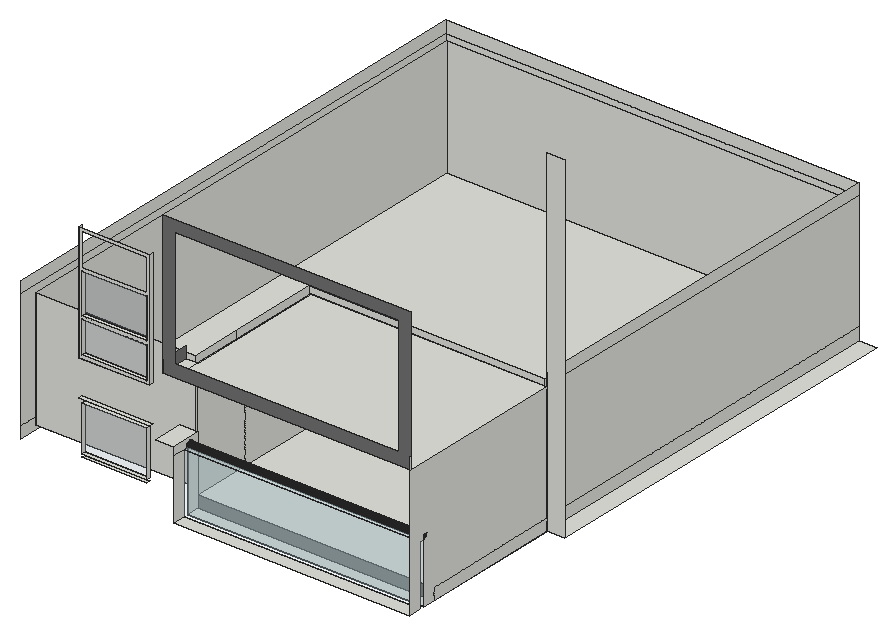
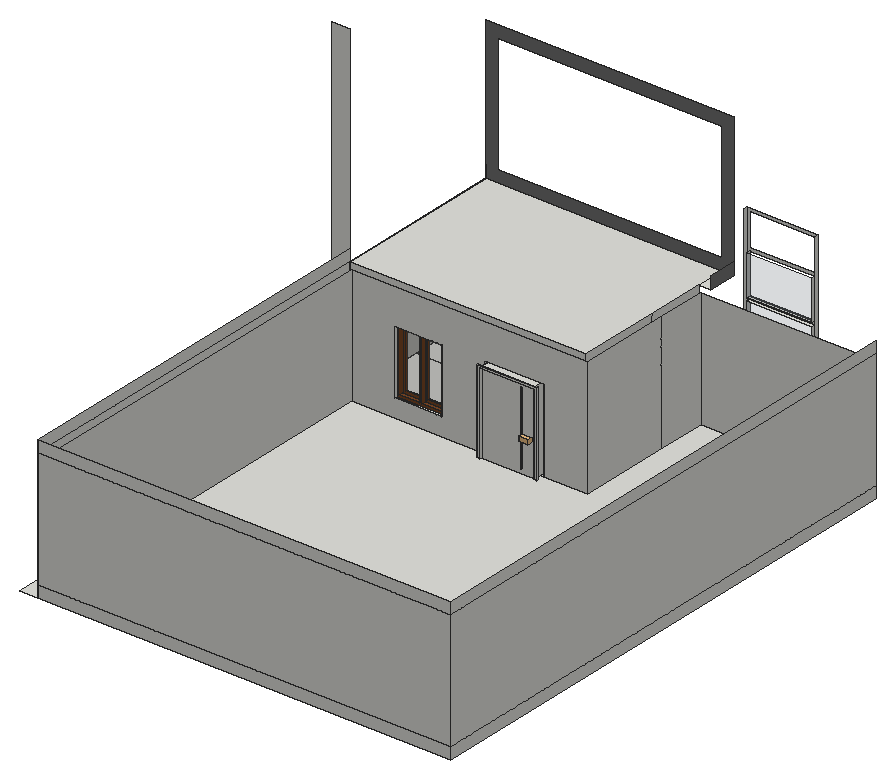
# SketchUp Ruby script. Lengths in inches.
U = 1.inch
M = Sketchup.active_model
def pt(a) = Geom::Point3d.new(a.map { |v| v * U })
def face(e, loops, mat)
  f = e.add_face(loops[0].map { |a| pt(a) })
  loops[1..].each { |l| e.add_face(l.map { |a| pt(a) }).erase! }
  f.material = f.back_material = mat if mat
  f
end
# faces: each face lists its corners as indices into pts; further lists are holes
def faces(e, pts, list, mat = nil) = list.each { |f| face(e, (f[0].is_a?(Array) ? f : [f]).map { |l| l.map { |i| pts[i] } }, mat) }
# xy, xz, yz: faces in a plane at the given z, y or x. An outline is a flat list of corners, or four numbers for a rectangle; further outlines are holes
def ring(l) = l.size == 4 ? [[l[0], l[1]], [l[2], l[1]], [l[2], l[3]], [l[0], l[3]]] : l.each_slice(2).to_a
def flat(e, list, mat, &to3) = list.each { |f| face(e, (f[0].is_a?(Array) ? f : [f]).map { |l| ring(l).map { |u, v| to3.(u, v) } }, mat) }
def xy(e, z, list, mat = nil) = flat(e, list, mat) { |x, y| [x, y, z] }
def xz(e, y, list, mat = nil) = flat(e, list, mat) { |x, z| [x, y, z] }
def yz(e, x, list, mat = nil) = flat(e, list, mat) { |y, z| [x, y, z] }
def lines(e, pts, list) = list.each { |a, b| e.add_line(pt(pts[a]), pt(pts[b])) }
# prism: a flat outline (further loops are holes) pulled along v
def prism(e, loops, v, mat = nil)
  f = face(e, loops, mat); d = Geom::Vector3d.new(v.map { |x| x * U })
  f.pushpull(f.normal.samedirection?(d) ? d.length : -d.length)
end
def box(e, o, s, mat = nil) = prism(e, [[o, [o[0] + s[0], o[1], o[2]], [o[0] + s[0], o[1] + s[1], o[2]], [o[0], o[1] + s[1], o[2]]]], [0, 0, s[2]], mat)
def at(x, y, z, deg = 0) = Geom::Transformation.translation(pt([x, y, z])) * Geom::Transformation.rotation(ORIGIN, Z_AXIS, deg.degrees)
def axes(o, x, y, z) = Geom::Transformation.new([*x, 0, *y, 0, *z, 0, *pt(o).to_a, 1])
def part(name) = M.definitions.add(name)
# library, detail: a bought-in or finely detailed component or shape, given as its bounding box
def library(name, o, s) = part(name).tap { |d| box(d.entities, o, s) }
def detail(e, o, s) = box(e.add_group.entities, o, s)
def put(e, d, t, mat = nil) = e.add_instance(d, t).tap { |i| i.material = mat if mat }
def group(e, t, mat = nil) = e.add_group.tap { |g| g.transformation = t; g.material = mat if mat }.entities
root = M.entities
M.materials.add("Glass_Basic_01").color = [161, 173, 186]
M.materials["Glass_Basic_01"].alpha = 0.25
M.materials.add("Glass_Safety_01").color = [204, 235, 244]
M.materials["Glass_Safety_01"].alpha = 0.25
M.materials.add("M05_Graphite_Haze").color = [114, 114, 114]
M.materials.add("Metal_06_1K").color = [238, 236, 231]
M.materials.add("[Translucent Glass Gray]").color = [132, 132, 132]
M.materials["[Translucent Glass Gray]"].alpha = 0.25
M.materials.add("[Wood Veneer 01]").color = [120, 70, 37]
c1 = part("Group\#8")
xy(c1.entities,0,[[0,0,19.69,1.18]],"[Wood Veneer 01]")
xy(c1.entities,2.76,[[2.76,0,16.93,1.18]],"[Wood Veneer 01]")
xy(c1.entities,60.24,[[2.76,0,16.93,1.18]],"[Wood Veneer 01]")
xy(c1.entities,62.99,[[0,0,19.69,1.18]],"[Wood Veneer 01]")
xz(c1.entities,0,[[2.76,2.76,16.93,60.24]],"[Translucent Glass Gray]")
xz(c1.entities,0,[[[0,0,19.69,62.99],[2.76,2.76,16.93,60.24]]],"[Wood Veneer 01]")
xz(c1.entities,1.18,[[[0,0,19.69,62.99],[2.76,2.76,16.93,60.24]]],"[Wood Veneer 01]")
yz(c1.entities,0,[[0,0,1.18,62.99]],"[Wood Veneer 01]")
yz(c1.entities,2.76,[[0,2.76,1.18,60.24]],"[Wood Veneer 01]")
yz(c1.entities,16.93,[[0,2.76,1.18,60.24]],"[Wood Veneer 01]")
yz(c1.entities,19.69,[[0,0,1.18,62.99]],"[Wood Veneer 01]")
c2 = part("pintu 2")
put(c2.entities,c1,at(-19.69,0,1.97))
g1 = group(c2.entities,at(-21.65,0,0))
prism(g1,[[[0,0,66.93],[0,0,0],[45.28,0,0],[45.28,0,66.93]],[[43.31,0,1.97],[23.62,0,1.97],[23.62,0,64.96],[43.31,0,64.96]],[[21.65,0,64.96],[21.65,0,1.97],[1.97,0,1.97],[1.97,0,64.96]]],[0,5.91,0],"[Wood Veneer 01]")
put(c2.entities,c1,at(1.97,0,1.97))
c3 = library("CLASSIC-BRASS_CHAUTAUQUA_LEVER-HARDWARE",[7.77,-2.58,0],[5.5,6.97,4.76])
xy(root,144,[[271.5,47.44,511.5,60.19],[271.5,64.66,511.5,77.44],[271.5,77.44,511.5,221.44],[511.5,221.87,529.5,617.44]])
xy(root,152.13,[[157.5,73.44,223.5,77.44]])
xy(root,155,[[157.5,73.44,223.5,77.44]])
xy(root,156,[[271.5,77.44,511.5,137.44],[100.5,86.44,262.5,86.44,262.5,230.44,310.875,230.44,310.875,233.83,310.2,233.83,310.2,237.47,307.5,237.47,307.5,238.93,310.875,238.93,310.875,233.83,311.21,233.83,311.21,237.47,364.86,237.47,364.86,238.93,368.23,238.93,368.23,237.47,365.53,237.47,365.53,233.83,364.86,233.83,364.86,230.44,502.5,230.44,502.5,608.44,100.5,608.44],[271.5,137.44,511.5,137.44,511.5,221.44,364.86,221.44,364.86,222.9,364.52,222.9,364.52,230.44,311.21,230.44,311.21,222.9,310.875,222.9,310.875,221.44,271.5,221.44],[307.5,221.44,310.875,222.9],[364.86,221.44,367.5,222.9],
  [367.5,221.44,368.23,222.9],[307.5,222.9,310.875,230.44],[310.875,222.9,311.21,230.44],[364.52,222.9,364.86,230.44],[364.86,222.9,367.5,230.44],
  [310.875,230.44,311.21,230.44,311.21,233.83,310.875,233.83,310.875,237.47,310.2,237.47,310.2,233.83,310.875,233.83],[311.21,230.44,364.52,233.83],[364.52,230.44,364.86,231.64],[364.52,231.64,364.86,231.64,364.86,233.83,365.2,233.83,365.2,237.47,364.86,237.47,364.86,233.83,364.52,233.83],[311.21,233.83,364.86,237.47],
  [365.2,233.83,365.53,237.47],[307.5,237.47,310.875,238.93],[364.86,237.47,368.23,238.93]])
xy(root,159.82,[[324.03,233.83,324.71,234.56],[324.03,236.75,324.71,237.47]])
xy(root,174.39,[[410.69,221.44,458.69,230.44]])
xy(root,202.13,[[157.5,73.44,223.5,77.44]])
xy(root,205.13,[[154.5,73.44,226.5,77.44]])
xy(root,205.15,[[271.5,60.19,511.5,64.66]],"Glass_Safety_01")
xy(root,213.3,[[253.5,47.44,271.5,77.44]])
xy(root,234.27,[[324.03,233.83,324.71,234.56],[324.03,236.75,324.71,237.47]])
xy(root,237.9,[[311.21,222.9,364.52,233.83]])
xy(root,238.09,[[310.875,221.44,364.86,222.9],[364.52,222.9,364.86,231.64],[310.2,233.83,310.875,237.47],[310.875,233.83,311.21,237.47],[311.21,233.83,364.86,237.47],
  [364.86,233.83,365.2,237.47],[365.2,233.83,365.53,237.47],[310.875,237.47,364.86,238.93]])
xy(root,239.43,[[310.875,222.9,364.86,237.47]])
xy(root,240,[[307.5,221.44,367.5,222.9],[367.5,221.44,368.23,222.9],[410.69,221.44,458.69,230.44],[307.5,222.9,367.5,230.44],[307.5,237.47,368.23,238.93]])
xy(root,242.1,[[154.5,73.44,226.5,77.44]])
xy(root,245.1,[[157.5,73.44,223.5,77.44]])
xy(root,276,[[259.5,48.44,271.5,77.44],[271.5,48.44,511.5,221.44]])
xy(root,278.1,[[157.5,73.44,223.5,77.44]])
xy(root,281.1,[[157.5,73.44,223.5,77.44]])
xz(root,48.44,[[[259.5,276,511.5,420],[271.5,288,499.5,408]]],"M05_Graphite_Haze")
xz(root,60.19,[[271.5,144,511.5,205.15]],"Glass_Safety_01")
xz(root,64.66,[[271.5,144,511.5,205.15]],"Glass_Safety_01")
xz(root,73.44,[[[154.5,242.1,226.5,361.04],[157.5,281.1,223.5,322.04],[157.5,325.04,223.5,358.04],[157.5,245.1,223.5,278.1]]])
xz(root,77.44,[[157.5,155,223.5,202.13],[157.5,245.1,223.5,278.1],[157.5,281.1,223.5,322.04]],"Glass_Basic_01")
xz(root,77.44,[[271.5,144,511.5,156]],"M05_Graphite_Haze")
xz(root,86.44,[[100.5,156,262.5,276]])
xz(root,221.44,[[[271.5,156,307.5,156,307.5,240,368.23,240,368.23,156,511.5,156,511.5,276,271.5,276],[410.69,174.39,458.69,240]],[307.5,156,310.875,156,310.875,238.09,364.86,238.09,364.86,156,367.5,156,367.5,240,307.5,240],[367.5,156,368.23,240]])
xz(root,221.87,[[511.5,144,529.5,488.3125]])
xz(root,222.9,[[307.5,156,310.875,238.47],[310.875,156,311.21,238.09],[364.52,156,364.86,238.09],[364.86,156,368.23,238.47],[311.21,237.9,364.52,238.09],
  [310.875,238.09,364.86,239.43],[307.5,238.47,307.5,240,368.23,240,368.23,238.47,364.86,238.47,364.86,239.43,310.875,239.43,310.875,238.47]])
xz(root,230.44,[[[262.5,156,262.5,276,502.5,276,502.5,156,367.5,156,367.5,240,307.5,240,307.5,156],[410.69,174.39,458.69,240]]])
xz(root,233.83,[[310.2,156,310.875,238.09],[310.875,156,311.21,237.9],[[311.21,156,364.52,237.9],[324.03,159.82,324.71,234.27]],[364.52,156,364.86,237.9],[364.86,156,365.2,238.09],
  [365.2,156,365.53,238.09],[310.875,237.9,311.21,238.09],[311.21,237.9,364.86,238.09]])
xz(root,234.56,[[324.03,159.82,324.71,234.27]])
xz(root,236.75,[[324.03,159.82,324.71,234.27]])
xz(root,237.47,[[307.5,156,310.2,156,310.2,238.09,310.875,238.09,310.875,238.47,307.5,238.47],[310.2,156,310.875,238.09],[[311.21,156,364.86,238.09],[324.03,159.82,324.71,234.27]],[364.86,156,365.2,238.09],[365.53,156,368.23,156,368.23,238.47,364.86,238.47,364.86,238.09,365.53,238.09],
  [365.2,156,365.53,238.09],[310.875,238.09,364.86,239.43],[307.5,238.47,310.875,238.47,310.875,239.43,364.86,239.43,364.86,238.47,368.23,238.47,368.23,240,307.5,240]])
xz(root,238.93,[[307.5,156,307.5,240,368.23,240,368.23,156,364.86,156,364.86,238.09,310.875,238.09,310.875,156]])
xz(root,608.44,[[100.5,156,502.5,276]])
xz(root,617.44,[[91.5,144,511.5,156],[91.5,156,511.5,276],[91.5,276,511.5,288]])
yz(root,91.5,[[77.44,144,617.44,156],[77.44,156,617.44,276],[77.44,276,617.44,288]])
yz(root,100.5,[[86.44,156,608.44,276]])
yz(root,154.5,[[73.44,242.1,77.44,361.04]])
yz(root,157.5,[[73.44,155,77.44,202.13],[73.44,245.1,77.44,278.1],[73.44,281.1,77.44,322.04]])
yz(root,223.5,[[73.44,155,77.44,202.13],[73.44,245.1,77.44,278.1],[73.44,281.1,77.44,322.04]])
yz(root,226.5,[[73.44,242.1,77.44,361.04]])
yz(root,259.5,[[48.44,276,77.44,288]],"M05_Graphite_Haze")
yz(root,262.5,[[86.44,156,137.44,276],[137.44,156,230.44,276]])
yz(root,271.5,[[47.44,144,60.19,205.15],[65.94,144,77.44,144,77.44,213.3,47.44,213.3,47.44,205.15,60.19,205.15,60.19,205.26,64.66,205.26,64.04,205.74,63.57,206.35,63.27,207.07,63.17,207.84,63.27,208.61,63.57,209.33,64.04,209.95,64.66,210.42,65.375,210.72,66.15,210.82,66.92,210.72,67.64,210.42,68.25,209.95,68.73,209.33,69.02,208.61,69.125,207.84,69.02,207.07,68.73,206.35,68.25,205.74,67.64,205.26,66.92,204.96,66.15,204.86,65.94,204.89],[64.66,144,65.94,144,65.94,204.89,65.375,204.96,64.92,205.15,64.66,205.15],[77.44,156,137.44,276],[137.44,156,221.44,276],
  [66.15,204.86,65.94,204.89,65.94,205.15,64.92,205.15,64.66,205.26,64.04,205.74,63.57,206.35,63.27,207.07,63.17,207.84,63.27,208.61,63.57,209.33,64.04,209.95,64.66,210.42,65.375,210.72,66.15,210.82,66.92,210.72,67.64,210.42,68.25,209.95,68.73,209.33,69.02,208.61,69.125,207.84,69.02,207.07,68.73,206.35,68.25,205.74,67.64,205.26,66.92,204.96],[65.94,204.89,65.375,204.96,64.92,205.15,65.94,205.15],[60.19,205.15,64.66,205.26],[64.66,205.15,64.92,205.15,64.66,205.26]])
yz(root,307.5,[[221.44,156,222.9,240],[222.9,156,230.44,240],[237.47,156,238.93,240]])
yz(root,310.2,[[233.83,156,237.47,238.09]])
yz(root,310.875,[[221.44,156,222.9,238.09],[222.9,156,222.9,239.43,237.47,239.43,237.47,238.09,233.83,238.09,233.83,156],[233.83,156,237.47,237.9],[237.47,156,238.93,238.09],[233.83,237.9,237.47,238.09]])
yz(root,311.21,[[222.9,156,233.83,237.9],[233.83,156,237.47,238.09]])
yz(root,324.03,[[233.83,159.82,234.56,234.27],[236.75,159.82,237.47,234.27]])
yz(root,324.71,[[233.83,159.82,234.56,234.27],[236.75,159.82,237.47,234.27]])
yz(root,364.52,[[222.9,156,233.83,237.9],[222.9,237.9,231.64,238.09]])
yz(root,364.86,[[221.44,156,222.9,238.09],[222.9,156,231.64,238.09],[231.64,156,233.83,156,233.83,238.09,237.47,238.09,237.47,239.43,222.9,239.43,222.9,238.09,231.64,238.09],[233.83,156,237.47,237.9],[237.47,156,238.93,238.09],
  [233.83,237.9,237.47,238.09]])
yz(root,365.2,[[233.83,156,237.47,238.09]])
yz(root,365.53,[[233.83,156,237.47,238.09]])
yz(root,367.5,[[221.44,156,230.44,240]])
yz(root,368.23,[[221.44,156,222.9,240],[237.47,156,238.93,240]])
yz(root,410.69,[[221.44,174.39,230.44,240]])
yz(root,458.69,[[221.44,174.39,230.44,240]])
yz(root,502.5,[[230.44,156,608.44,276]])
yz(root,511.5,[[[47.44,144,47.44,276,221.44,276,221.44,156,77.44,156,77.44,144,64.66,144,64.66,205.15,60.19,205.15,60.19,144],[66.15,204.86,66.92,204.96,67.64,205.26,68.25,205.74,68.73,206.35,69.02,207.07,69.125,207.84,69.02,208.61,68.73,209.33,68.25,209.95,67.64,210.42,66.92,210.72,66.15,210.82,65.375,210.72,64.66,210.42,64.04,209.95,63.57,209.33,63.27,208.61,63.17,207.84,63.27,207.07,63.57,206.35,64.04,205.74,64.66,205.26,65.375,204.96]],[77.44,144,221.87,156],[221.87,144,617.44,156],[221.44,156,221.87,276],[221.87,156,617.44,276],
  [47.44,276,48.44,288],[221.87,276,617.44,288]])
p = [[271.5,65.375,204.96],[271.5,65.94,204.89],[271.5,66.15,204.86],[511.5,66.15,204.86],[511.5,65.375,204.96],[271.5,66.92,204.96],
  [511.5,66.92,204.96],[271.5,64.66,205.26],[271.5,64.92,205.15],[511.5,64.66,205.26],[271.5,67.64,205.26],[511.5,67.64,205.26],
  [271.5,64.04,205.74],[511.5,64.04,205.74],[271.5,68.25,205.74],[511.5,68.25,205.74],[271.5,63.57,206.35],[511.5,63.57,206.35],
  [271.5,68.73,206.35],[511.5,68.73,206.35],[271.5,63.27,207.07],[511.5,63.27,207.07],[271.5,69.02,207.07],[511.5,69.02,207.07],
  [271.5,63.17,207.84],[511.5,63.17,207.84],[271.5,69.125,207.84],[511.5,69.125,207.84],[271.5,63.27,208.61],[511.5,63.27,208.61],
  [271.5,69.02,208.61],[511.5,69.02,208.61],[271.5,63.57,209.33],[511.5,63.57,209.33],[271.5,68.73,209.33],[511.5,68.73,209.33],
  [271.5,64.04,209.95],[511.5,64.04,209.95],[271.5,68.25,209.95],[511.5,68.25,209.95],[271.5,64.66,210.42],[511.5,64.66,210.42],
  [271.5,67.64,210.42],[511.5,67.64,210.42],[271.5,65.375,210.72],[511.5,65.375,210.72],[271.5,66.92,210.72],[511.5,66.92,210.72],
  [271.5,66.15,210.82],[511.5,66.15,210.82],[271.5,66.15,207.84],[511.5,66.15,207.84]]
faces(root,p,[[0,1,2,3,4],[2,5,6,3],[7,8,0,4,9],[5,10,11,6],[12,7,9,13],[10,14,15,11],[16,12,13,17],[14,18,19,15],
  [20,16,17,21],[18,22,23,19],[24,20,21,25],[22,26,27,23],[28,24,25,29],[26,30,31,27],[32,28,29,33],[30,34,35,31],
  [36,32,33,37],[34,38,39,35],[40,36,37,41],[38,42,43,39],[44,40,41,45],[42,46,47,43],[48,44,45,49],[46,48,49,47]],"Metal_06_1K")
lines(root,p,[[50,51]])
put(root,c2,axes([433.65,221.44,174.39],[1.06017,0,0],[0,1,0],[0,0,0.98046]))
put(root,c3,axes([336.84,237.33,192.3],[-1.71399,0,0],[0,-1.8508,0],[0,0,-0.96982]))
